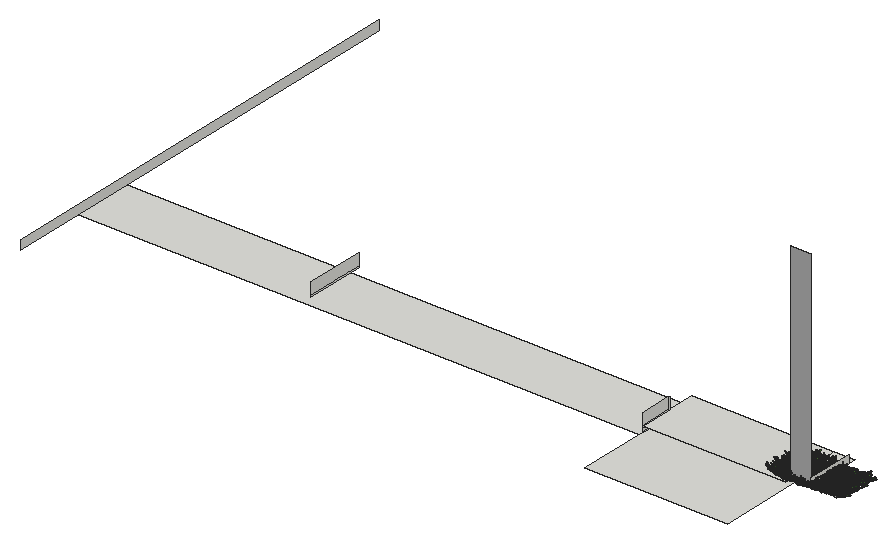
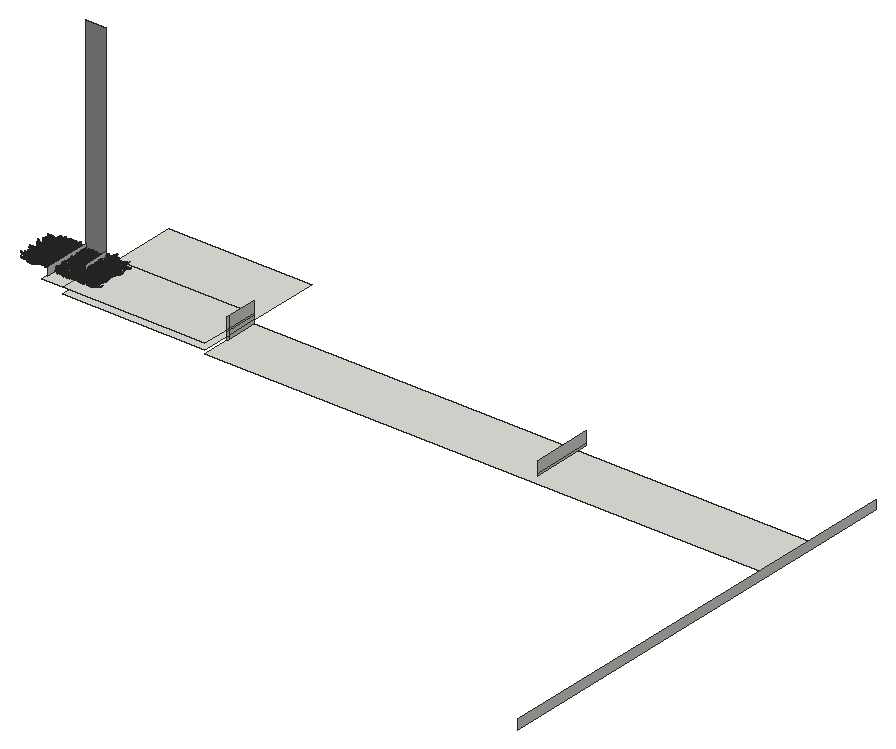
# SketchUp Ruby script. Lengths in inches.
U = 1.inch
M = Sketchup.active_model
def pt(a) = Geom::Point3d.new(a.map { |v| v * U })
def face(e, loops, mat)
  f = e.add_face(loops[0].map { |a| pt(a) })
  loops[1..].each { |l| e.add_face(l.map { |a| pt(a) }).erase! }
  f.material = f.back_material = mat if mat
  f
end
# faces: each face lists its corners as indices into pts; further lists are holes
def faces(e, pts, list, mat = nil) = list.each { |f| face(e, (f[0].is_a?(Array) ? f : [f]).map { |l| l.map { |i| pts[i] } }, mat) }
# xy, xz, yz: faces in a plane at the given z, y or x. An outline is a flat list of corners, or four numbers for a rectangle; further outlines are holes
def ring(l) = l.size == 4 ? [[l[0], l[1]], [l[2], l[1]], [l[2], l[3]], [l[0], l[3]]] : l.each_slice(2).to_a
def flat(e, list, mat, &to3) = list.each { |f| face(e, (f[0].is_a?(Array) ? f : [f]).map { |l| ring(l).map { |u, v| to3.(u, v) } }, mat) }
def xy(e, z, list, mat = nil) = flat(e, list, mat) { |x, y| [x, y, z] }
def xz(e, y, list, mat = nil) = flat(e, list, mat) { |x, z| [x, y, z] }
def yz(e, x, list, mat = nil) = flat(e, list, mat) { |y, z| [x, y, z] }
def lines(e, pts, list) = list.each { |a, b| e.add_line(pt(pts[a]), pt(pts[b])) }
# prism: a flat outline (further loops are holes) pulled along v
def prism(e, loops, v, mat = nil)
  f = face(e, loops, mat); d = Geom::Vector3d.new(v.map { |x| x * U })
  f.pushpull(f.normal.samedirection?(d) ? d.length : -d.length)
end
def box(e, o, s, mat = nil) = prism(e, [[o, [o[0] + s[0], o[1], o[2]], [o[0] + s[0], o[1] + s[1], o[2]], [o[0], o[1] + s[1], o[2]]]], [0, 0, s[2]], mat)
def at(x, y, z, deg = 0) = Geom::Transformation.translation(pt([x, y, z])) * Geom::Transformation.rotation(ORIGIN, Z_AXIS, deg.degrees)
def axes(o, x, y, z) = Geom::Transformation.new([*x, 0, *y, 0, *z, 0, *pt(o).to_a, 1])
def part(name) = M.definitions.add(name)
# library, detail: a bought-in or finely detailed component or shape, given as its bounding box
def library(name, o, s) = part(name).tap { |d| box(d.entities, o, s) }
def detail(e, o, s) = box(e.add_group.entities, o, s)
def put(e, d, t, mat = nil) = e.add_instance(d, t).tap { |i| i.material = mat if mat }
def group(e, t, mat = nil) = e.add_group.tap { |g| g.transformation = t; g.material = mat if mat }.entities
root = M.entities
M.materials.add("Material82").color = [68, 110, 58]
M.materials.add("Material83").color = [48, 90, 38]
M.materials.add("Material84").color = [68, 110, 48]
M.materials.add("Material85").color = [48, 90, 48]
M.materials.add("Material86").color = [58, 110, 58]
M.materials.add("Material87").color = [58, 90, 38]
M.materials.add("Material88").color = [68, 100, 58]
M.materials.add("Material89").color = [48, 100, 38]
M.materials.add("[Color M03]1").color = [170, 170, 170]
c1 = part("grass00")
p = [[-0.6875,0.15,0],[-0.56,0.08,5.52],[-0.04,0.03,2.76],[0.48,-0.02,0],[0.35,-0.02,5.52],[-0.1,-0.14,5.52],
  [-0.12,0.65,8.37],[-0.42,0.65,8.37]]
faces(c1.entities,p,[[0,1,2,3],[3,2,4],[1,5,2],[5,4,2],[1,6,5],[4,5,6],[7,6,1]])
c2 = part("Group16\#1")
put(c2.entities,c1,axes([1.44,-0.61,-0.01],[0.05352,0.12609,0],[-0.10704,0.04543,0.07239],[0.06664,-0.02828,0.11628]),"Material85")
put(c2.entities,c1,axes([0.76,-0.15,-0.01],[0.04676,0.24062,0],[-0.23162,0.04501,0.06642],[0.0652,-0.01267,0.23595]),"Material82")
put(c2.entities,c1,axes([0.79,0.01,-0.01],[-0.00606,0.34651,0],[-0.34381,-0.00602,0.0432],[0.04319,0.00076,0.34386]))
put(c2.entities,c1,axes([1,0.23,-0.01],[-0.07192,0.31144,0],[-0.28722,-0.06632,0.1236],[0.12043,0.02781,0.29478]),"Material84")
put(c2.entities,c1,axes([1.66,0.77,-0.01],[-0.13828,0.29651,0],[-0.21551,-0.1005,0.22471],[0.20365,0.09498,0.23779]),"Material89")
put(c2.entities,c1,axes([0.6875,0.52,-0.01],[-0.18126,0.24051,0],[-0.22746,-0.17142,0.09788],[0.07817,0.05891,0.28481]),"Material84")
put(c2.entities,c1,axes([0.68,0.78,-0.01],[-0.215,0.18688,0],[-0.12385,-0.14248,0.21334],[0.13995,0.16101,0.18878]),"Material82")
put(c2.entities,c1,axes([0.56,1,-0.01],[-0.13756,0.07624,0],[-0.06159,-0.11112,0.0927],[0.04494,0.08108,0.12705]),"Material84")
put(c2.entities,c1,axes([0.2,0.64,-0.01],[-0.23729,0.07254,0],[-0.05711,-0.18681,0.153],[0.04473,0.14632,0.19535]),"Material89")
put(c2.entities,c1,axes([0.0625,0.72,-0.01],[-0.28874,0.02525,0],[-0.02179,-0.24916,0.14647],[0.01276,0.14591,0.25012]),"Material82")
put(c2.entities,c1,axes([-0.08,0.62,-0.01],[-0.34089,-0.04187,0],[0.03255,-0.26504,0.216],[-0.02633,0.21439,0.26703]),"Material89")
put(c2.entities,c1,axes([-0.34,0.98,-0.01],[-0.14314,-0.0493,0],[0.04397,-0.12769,0.06843],[-0.02228,0.0647,0.13505]),"Material89")
put(c2.entities,c1,axes([-0.87,1.45,-0.01],[-0.23488,-0.14114,0],[0.13761,-0.22901,0.06087],[-0.03135,0.05217,0.26717]))
put(c2.entities,c1,axes([-0.72,0.77,-0.01],[-0.14208,-0.13251,0],[0.07209,-0.0773,0.16301],[-0.11118,0.11922,0.1057]),"Material89")
put(c2.entities,c1,axes([-0.62,0.43,-0.01],[-0.14845,-0.21203,0],[0.18654,-0.13061,0.12304],[-0.10079,0.07057,0.22772]),"Material82")
put(c2.entities,c1,axes([-0.68,0.29,-0.01],[-0.13639,-0.32136,0],[0.31723,-0.13464,0.05579],[-0.05136,0.0218,0.34462]),"Material83")
put(c2.entities,c1,axes([-0.64,0.125,-0.01],[-0.0458,-0.23569,0],[0.22124,-0.043,0.08276],[-0.08124,0.01579,0.22538]),"Material86")
put(c2.entities,c1,axes([-1.6,-0.03,-0.01],[0.00576,-0.32897,0],[0.27526,0.00482,0.18018],[-0.18015,-0.00315,0.2753]),"Material84")
put(c2.entities,c1,axes([-1.36,-0.31,-0.01],[0.05718,-0.24765,0],[0.18172,0.04196,0.17267],[-0.16825,-0.03885,0.1865]),"Material89")
put(c2.entities,c1,axes([-1.54,-0.72,-0.01],[0.06537,-0.14017,0],[0.13555,0.06321,0.03939],[-0.0357,-0.01665,0.14956]))
put(c2.entities,c1,axes([-1.19,-0.9,-0.01],[0.09597,-0.12735,0],[0.11214,0.08451,0.07557],[-0.06035,-0.04548,0.14042]),"Material88")
put(c2.entities,c1,axes([-0.47,-0.54,-0.01],[0.11588,-0.10072,0],[0.0618,0.0711,0.12124],[-0.07953,-0.0915,0.0942]))
put(c2.entities,c1,axes([-0.47,-0.84,-0.01],[0.11927,-0.0661,0],[0.06603,0.11913,0.00646],[-0.00313,-0.00565,0.13621]),"Material84")
put(c2.entities,c1,axes([-0.38,-1.24,-0.01],[0.28037,-0.08571,0],[0.0618,0.20215,0.20315],[-0.05939,-0.19428,0.21139]),"Material88")
put(c2.entities,c1,axes([-0.06,-0.66,-0.01],[0.22719,-0.01987,0],[0.01247,0.14255,0.17758],[-0.01547,-0.17691,0.1431]),"Material87")
put(c2.entities,c1,axes([0.11,-0.89,-0.01],[0.14882,0.01828,0],[-0.01058,0.08611,0.12229],[0.01491,-0.12138,0.08676]),"Material85")
put(c2.entities,c1,axes([0.25,-0.72,-0.01],[0.20481,0.07053,0],[-0.06206,0.18022,0.10291],[0.03351,-0.0973,0.1906]),"Material85")
put(c2.entities,c1,axes([0.85,-1.42,-0.01],[0.16481,0.09904,0],[-0.09472,0.15762,0.05616],[0.02893,-0.04814,0.18389]),"Material84")
put(c2.entities,c1,axes([1.01,-1.09,-0.01],[0.21858,0.20385,0],[-0.17495,0.1876,0.15339],[0.10462,-0.11218,0.25652]),"Material89")
put(c2.entities,c1,axes([1.01,-0.71,-0.01],[0.08733,0.12473,0],[-0.06445,0.04512,0.13037],[0.1068,-0.07477,0.07867]),"Material85")
c3 = part("Group15\#1")
put(c3.entities,c2,at(0,0,0))
c4 = part("3darcstudiotree_grass00\#1")
put(c4.entities,c3,at(0,0,0))
xy(root,-42.1875,[[0.34,335.84,486.41,387.84]])
xy(root,-39.125,[[486.41,273.41,609.09,387.84]])
xy(root,-34.17,[[486.41,335.84,609.09,387.84],[609.09,341.03,626.68,387.84]])
xz(root,341.03,[[609.09,-34.17,626.68,144.9375]],"[Color M03]1")
yz(root,0.34,[[273.41,-42.1875,273.41,-38.0625,273.53,-38.0625,273.53,-34.17,659.09,-34.17,659.09,-42.1875]])
yz(root,200.03,[[335.84,-35.625,387.84,-34.17],[335.84,-34.17,387.84,-24.25]])
yz(root,486.41,[[335.84,-42.1875,362.97,-39.125],[362.97,-42.1875,364.46,-39.125],[335.84,-39.125,362.97,-35.625],[362.97,-39.125,364.46,-35.625],[335.84,-35.625,362.97,-34.17],
  [362.97,-35.625,364.46,-34.17],[335.84,-34.17,362.97,-24.25],[362.97,-34.17,364.46,-24.25]])
yz(root,609.09,[[341.03,-34.17,362.97,-27.66]])
yz(root,626.68,[[341.03,-34.17,381.72,-27.66]])
put(root,c4,axes([596.77,350.95,-34.17],[-3.06097,-0.5879,0],[1.66705,-1.34995,-0.03924],[0.1162,-0.0941,1.93013]))
put(root,c4,axes([597.85,372.86,-34.17],[0.43217,-1.5656,0],[4.20709,0.18062,-0.01362],[0.0661,0.00284,1.54899]))
put(root,c4,axes([598.34,355.5625,-34.17],[-4.03652,-0.16228,0],[0.44348,-1.71564,-0.03002],[0.01485,-0.05745,1.59842]))
put(root,c4,axes([598.04,360.35,-34.17],[2.89762,-1.1399,0],[2.43274,0.96179,-0.0036],[0.01556,0.00615,1.5794]))
put(root,c4,axes([597.95,342.71,-34.17],[3.9501,-0.3019,0],[0.82816,1.68526,-0.01483],[0.01308,0.02661,1.51152]))
put(root,c4,axes([597.65,364.46,-34.17],[3.35543,0.83331,0],[-2.02345,1.2672,-0.03908],[-0.13338,0.08353,1.82303]))
put(root,c4,axes([598.39,348.62,-34.17],[2.855,1.42821,0],[-2.79418,0.86872,-0.04305],[-0.19263,0.05989,1.51958]))
put(root,c4,axes([600.08,371.03,-34.17],[4.14496,0.31804,0],[-0.83759,1.6978,-0.03864],[-0.04159,0.0843,1.85268]))
put(root,c4,axes([600.26,342.22,-34.17],[3.14768,1.20624,0],[-3.13864,1.27383,-0.06236],[-0.23969,0.09728,1.86199]))
put(root,c4,axes([601.58,367.78,-34.17],[1.22629,-1.22817,0],[3.78204,0.58732,-0.0431],[0.18193,0.02825,1.38217]))
put(root,c4,axes([601.63,354.84,-34.17],[2.09831,-1.02697,0],[3.53268,1.1226,-0.04335],[0.15343,0.04876,1.54559]))
put(root,c4,axes([601.5,351.3,-34.17],[-2.72452,1.24598,0],[-3.55259,-1.2082,-0.04683],[-0.18808,-0.06396,1.86493]))
put(root,c4,axes([600.98,357.3125,-34.17],[3.77194,0.53127,0],[-1.56854,1.73204,-0.02984],[-0.04464,0.0493,1.55474]))
put(root,c4,axes([602.62,353.18,-34.17],[0.71144,-1.32945,0],[4.31841,0.35942,-0.04294],[0.17046,0.01419,1.34209]))
put(root,c4,axes([602.9,360.26,-34.17],[1.7149,-1.22637,0],[3.67075,0.79833,-0.00061],[0.00329,0.00072,1.94394]))
put(root,c4,axes([603.23,362.27,-34.17],[1.13517,-1.33714,0],[4.08386,0.53922,-0.04023],[0.16123,0.02129,1.36415]))
put(root,c4,axes([602.3125,366.27,-34.17],[-1.96155,1.42232,0],[-3.86474,-0.82896,-0.01158],[-0.04562,-0.00979,1.47884]))
put(root,c4,axes([603.71,372.46,-34.17],[-0.47401,-1.83018,0],[3.81106,-0.15352,-0.01024],[0.06486,-0.00261,1.82793]))
put(root,c4,axes([603.14,363.91,-34.17],[-2.22727,1.60419,0],[-4.12877,-0.89155,-0.00813],[-0.02667,-0.00576,1.31962]))
put(root,c4,axes([603.48,348.36,-34.17],[-2.60888,1.40075,0],[-3.4553,-1.0009,-0.02364],[-0.11495,-0.0333,1.93862]))
put(root,c4,axes([603.86,347.26,-34.17],[3.43972,-1.19732,0],[3.07284,1.37298,-0.00351],[0.01073,0.00479,1.60808]))
put(root,c4,axes([603.88,344.94,-34.17],[2.57433,-1.10368,0],[3.03991,1.10279,-0.05921],[0.27011,0.09799,1.91907]))
put(root,c4,axes([605.8,364.41,-34.17],[-1.00872,-1.50256,0],[3.76018,-0.39261,-0.00114],[0.00668,-0.0007,1.77079]))
put(root,c4,axes([606.1,351.03,-34.17],[-4.39065,-0.68044,0],[1.48247,-1.48779,-0.03326],[0.06181,-0.06203,1.54402]))
put(root,c4,axes([606.08,365.79,-34.17],[-4.44259,0.07323,0],[-0.15396,-1.45277,-0.02048],[-0.00618,-0.05831,1.99696]))
put(root,c4,axes([605.59,361.58,-34.17],[-2.76199,0.84111,0],[-2.40625,-1.22891,-0.02049],[-0.06035,-0.03082,1.42185]))
put(root,c4,axes([606.19,344.48,-34.17],[4.22079,-0.16227,0],[0.44484,1.79962,-0.00515],[0.00263,0.01065,1.80879]))
put(root,c4,axes([608.31,341.46,-34.17],[-4.16244,-0.15093,0],[0.36502,-1.56574,-0.01686],[0.00714,-0.03063,1.38194]))
put(root,c4,axes([606.99,358.125,-34.17],[-0.6643,1.32662,0],[-4.47997,-0.3489,-0.01512],[-0.08059,-0.00628,1.85999]))
put(root,c4,axes([608.55,349.27,-34.17],[0.943,-1.41783,0],[3.80413,0.39351,-0.01105],[0.05525,0.00572,1.52421]))
put(root,c4,axes([607.11,340.13,-34.17],[0.93193,1.68006,0],[-3.63506,0.3136,-0.00261],[-0.01526,0.00132,1.6704]))
put(root,c4,axes([609.1875,355.56,-34.17],[-3.93808,-0.75827,0],[2.05575,-1.66052,-0.06565],[0.13947,-0.11266,1.70067]))
put(root,c4,axes([607.58,359.26,-34.17],[-0.07538,1.68656,0],[-4.43832,-0.03085,-0.00958],[-0.0427,-0.0003,1.48335]))
put(root,c4,axes([608.42,347.11,-34.17],[0.31598,1.50106,0],[-3.48689,0.11416,-0.00998],[-0.05116,0.00168,1.34846]))
put(root,c4,axes([609.24,371.18,-34.17],[3.02082,-1.15648,0],[2.42176,0.98385,-0.02978],[0.11407,0.04634,1.43312]))
put(root,c4,axes([608.69,367.64,-34.17],[3.58704,0.55594,0],[-1.39662,1.40151,-0.02634],[-0.05335,0.05353,1.58474]))
put(root,c4,axes([609.32,352.21,-34.17],[3.13564,-0.95157,0],[2.13614,1.09478,-0.03629],[0.11919,0.06109,1.41389]))
put(root,c4,axes([611.19,369.84,-34.17],[-3.8239,-0.32025,0],[0.87863,-1.63166,-0.02543],[0.02678,-0.04974,1.60712]))
put(root,c4,axes([611.99,364.32,-34.17],[-1.37854,-1.47975,0],[3.2131,-0.46555,-0.02344],[0.115,-0.01666,1.34096]))
put(root,c4,axes([611.77,346.58,-34.17],[-3.58928,0.33039,0],[-0.75882,-1.28211,-0.0198],[-0.02657,-0.04489,1.47686]))
put(root,c4,axes([611.6,366.04,-34.17],[1.03001,-1.55898,0],[3.46185,0.35573,-0.04641],[0.24674,0.02535,1.47323]))
put(root,c4,axes([612.35,361.51,-34.17],[0.07037,-1.71405,0],[4.70144,0.03002,-0.02796],[0.12644,0.00081,1.59394]))
put(root,c4,axes([612.45,358.96,-34.17],[-4.25189,0.62806,0],[-1.17044,-1.23238,-0.01358],[-0.02814,-0.02963,1.47772]))
put(root,c4,axes([612.82,357.41,-34.17],[-4.15804,-0.01553,0],[0.04454,-1.85443,-0.04475],[0.00172,-0.0718,1.43393]))
put(root,c4,axes([612.16,373.13,-34.17],[2.99211,-0.88341,0],[2.54027,1.33816,-0.01707],[0.06311,0.03325,1.96039]))
put(root,c4,axes([613.01,355.67,-34.17],[-3.68076,-0.30441,0],[0.87866,-1.65237,-0.00999],[0.00884,-0.01661,1.38276]))
put(root,c4,axes([612.66,369.11,-34.17],[-2.36198,1.34531,0],[-2.91809,-0.79683,-0.03104],[-0.17128,-0.04677,1.78553]))
put(root,c4,axes([613.125,344.33,-34.17],[2.97125,-1.188,0],[2.63587,1.02532,-0.00165],[0.00768,0.00299,1.81884]))
put(root,c4,axes([614.28,341.39,-34.17],[-4.35861,-0.14504,0],[0.36663,-1.71363,-0.02802],[0.01298,-0.06068,1.8014]))
put(root,c4,axes([612.98,352.64,-34.17],[3.6615,0.00284,0],[-0.00662,1.32579,-0.0306],[-0.00046,0.09111,1.9022]))
put(root,c4,axes([614.39,351.26,-34.17],[-3.40532,-0.07402,0],[0.22612,-1.61806,-0.00601],[0.00193,-0.01379,1.79325]))
put(root,c4,axes([613.38,349.14,-34.17],[3.15923,1.14894,0],[-3.00225,1.28393,-0.03053],[-0.12215,0.05224,1.95907]))
put(root,c4,axes([616.42,341.86,-34.17],[3.82244,-0.70635,0],[1.81239,1.52539,-0.00986],[0.01787,0.01504,1.36783]))
put(root,c4,axes([617.38,359.25,-34.17],[-3.50881,1.16011,0],[-2.69176,-1.26622,-0.04843],[-0.14054,-0.06611,1.41858]))
put(root,c4,axes([616.77,353.67,-34.17],[3.5983,-0.42057,0],[0.96573,1.28508,-0.03127],[0.05191,0.06908,1.48816]))
put(root,c4,axes([616.78,351.11,-34.17],[-1.39865,1.66077,0],[-3.78259,-0.49545,-0.00679],[-0.0282,-0.00369,1.30662]))
put(root,c4,axes([617.58,364.09,-34.17],[2.65926,-1.384,0],[3.07673,0.91944,-0.04967],[0.23773,0.07104,1.73743]))
put(root,c4,axes([616.96,346.05,-34.17],[3.23293,0.85538,0],[-2.19162,1.28829,-0.0468],[-0.14196,0.08345,1.60535]))
put(root,c4,axes([618.6875,373.03,-34.17],[0.37423,-1.77165,0],[3.6892,0.1212,-0.04948],[0.31334,0.01029,1.76318]))
put(root,c4,axes([618.08,370.58,-34.17],[-1.23102,1.43236,0],[-4.00109,-0.53481,-0.05878],[-0.24424,-0.03265,1.38915]))
put(root,c4,axes([619.35,368.61,-34.17],[-3.85586,-0.61181,0],[1.38378,-1.3564,-0.02256],[0.04705,-0.04612,1.55256]))
put(root,c4,axes([617.87,365.61,-34.17],[4.58666,-0.29954,0],[0.76961,1.83286,-0.06031],[0.05541,0.13196,1.9859]))
put(root,c4,axes([617.58,356.65,-34.17],[2.59618,1.43862,0],[-2.87173,0.80602,-0.01154],[-0.04691,0.01317,1.31865]))
put(root,c4,axes([619.11,344.33,-34.17],[0.50435,-1.60129,0],[3.80498,0.18639,-0.05019],[0.26525,0.01299,1.53052]))
put(root,c4,axes([618.4,362.3,-34.17],[3.24935,0.42764,0],[-1.43334,1.69386,-0.04175],[-0.05922,0.06999,1.52086]))
put(root,c4,axes([618.77,348.15,-34.17],[4.09406,-0.23131,0],[0.47213,1.29969,-0.032],[0.03631,0.09996,1.99674]))
put(root,c4,axes([619.21,340.25,-34.17],[1.78223,1.25772,0],[-3.10123,0.68348,-0.02391],[-0.11693,0.02577,1.49173]))
put(root,c4,axes([619.22,355.03,-34.17],[0.65139,1.7147,0],[-4.45072,0.26296,-0.01905],[-0.08769,0.00518,1.57029]))
put(root,c4,axes([622.5,370.89,-34.17],[-3.04991,-1.12114,0],[2.90905,-1.23081,-0.00052],[0.00199,-0.00084,1.79691]))
put(root,c4,axes([624.15,368.53,-34.17],[0.23876,-1.55199,0],[4.36064,0.10434,-0.04584],[0.18368,0.0044,1.3146]))
put(root,c4,axes([624.41,351.125,-34.17],[-0.00481,-1.55543,0],[4.64446,-0.00224,-0.02113],[0.08601,-0.00004,1.41674]))
put(root,c4,axes([623.08,344.05,-34.17],[3.47227,-0.30693,0],[0.74979,1.31925,-0.01015],[0.01336,0.0235,1.54623]))
put(root,c4,axes([623.05,346.05,-34.17],[-1.26342,1.38148,0],[-3.54227,-0.50384,-0.00809],[-0.04856,-0.00691,1.80065]))
put(root,c4,axes([623.6875,352.72,-34.17],[2.94151,-0.90679,0],[2.69176,1.35804,-0.00613],[0.02014,0.01016,1.74641]))
put(root,c4,axes([622.95,365.35,-34.17],[0.11831,1.37685,0],[-3.50344,0.04682,-0.00216],[-0.01444,0.00019,1.758]))
put(root,c4,axes([624.61,356.01,-34.17],[-0.73982,-1.44093,0],[3.74487,-0.29904,-0.04711],[0.2431,-0.01941,1.50792]))
put(root,c4,axes([624.1,361.35,-34.17],[2.48182,-1.04217,0],[2.75852,1.02169,-0.02466],[0.10108,0.03744,1.59511]))
put(root,c4,axes([623.93,348.7,-34.17],[-2.81085,1.01922,0],[-2.91901,-1.25203,-0.0061],[-0.02341,-0.01004,1.83281]))
put(root,c4,axes([623.87,341.63,-34.17],[-0.96185,1.4826,0],[-3.70839,-0.37418,-0.04208],[-0.21883,-0.02208,1.54007]))
put(root,c4,axes([625.34,359.52,-34.17],[-0.3225,-1.34219,0],[4.58247,-0.17125,-0.03587],[0.16603,-0.0062,1.60406]))
put(root,c4,axes([624.07,340.65,-34.17],[3.91343,0.66663,0],[-1.38696,1.26634,-0.02193],[-0.04877,0.04453,1.47013]))
put(root,c4,axes([624.88,363.84,-34.17],[3.82293,-1.07301,0],[2.00012,1.10831,-0.02041],[0.08948,0.04958,1.95445]))
put(root,c4,axes([624.75,357.49,-34.17],[3.70183,0.03147,0],[-0.07805,1.42775,-0.0399],[-0.00598,0.10931,1.8861]))
put(root,c4,axes([628.43,354.69,-34.17],[-0.79677,-1.6402,0],[3.36468,-0.25421,-0.01579],[0.08769,-0.00662,1.45182]))
put(root,c4,axes([628.94,350.28,-34.17],[-4.49567,-0.3985,0],[0.83225,-1.46029,-0.03373],[0.03467,-0.06083,1.33323]))
put(root,c4,axes([628.86,352.49,-34.17],[-4.6805,0.28538,0],[-0.54089,-1.37973,-0.03554],[-0.03758,-0.09587,1.83631]))
put(root,c4,axes([627.59,358.97,-34.17],[-0.10316,1.55622,0],[-4.09748,-0.04224,-0.03889],[-0.19104,-0.00197,1.50954]))
put(root,c4,axes([628.4,356.86,-34.17],[-3.29804,1.27107,0],[-2.52678,-1.01968,-0.01484],[-0.07094,-0.02863,1.85373]))
put(root,c4,axes([628.53,363.52,-34.17],[2.48968,-1.1461,0],[2.93182,0.99053,-0.00664],[0.0258,0.00872,1.48048]))
put(root,c4,axes([629.98,368.03,-34.17],[-1.20508,-1.27416,0],[3.97727,-0.58504,-0.0406],[0.22085,-0.03249,1.84742]))
put(root,c4,axes([629.125,346.98,-34.17],[-0.56456,1.41966,0],[-3.50259,-0.21664,-0.01794],[-0.10644,-0.00658,1.59592]))
put(root,c4,axes([629.1,366.93,-34.17],[1.96349,1.64722,0],[-3.56633,0.66117,-0.03464],[-0.18907,0.03505,1.78143]))
put(root,c4,axes([630.91,361.32,-34.17],[2.10633,-1.56652,0],[4.07545,0.85227,-0.05067],[0.19625,0.04104,1.51576]))
put(root,c4,axes([630.82,341.8,-34.17],[2.08347,-1.59715,0],[3.15506,0.64012,-0.03693],[0.21917,0.04447,1.77491]))
put(root,c4,axes([629.86,348.7,-34.17],[0.79004,1.45858,0],[-4.26548,0.35933,-0.00171],[-0.00893,0.00075,1.74655]))
put(root,c4,axes([631.58,371.06,-34.17],[1.69514,-1.26112,0],[3.85825,0.80658,-0.01977],[0.09529,0.01992,1.78562]))
put(root,c4,axes([630.44,343.68,-34.17],[3.33408,0.32893,0],[-1.10916,1.74856,-0.00744],[-0.00738,0.01164,1.4009]))
put(root,c4,axes([634.15,348.7,-34.17],[-4.09965,-0.15274,0],[0.36855,-1.53851,-0.03137],[0.01329,-0.05547,1.3228]))
put(root,c4,axes([633.6,366.12,-34.17],[-3.21191,1.28173,0],[-2.59769,-1.01243,-0.03007],[-0.15402,-0.06003,1.97134]))
put(root,c4,axes([634.6,356.73,-34.17],[-1.51918,-1.57572,0],[4.39344,-0.65879,-0.02869],[0.10716,-0.01607,1.40786]))
put(root,c4,axes([634.97,341.9,-34.17],[-4.22007,0.35003,0],[-0.86715,-1.62599,-0.01674],[-0.0198,-0.03713,1.81501]))
put(root,c4,axes([634.34,361.08,-34.17],[-1.69964,1.49974,0],[-3.25198,-0.57319,-0.0353],[-0.21623,-0.03811,1.79152]))
put(root,c4,axes([634.31,360.03,-34.17],[-1.65501,1.23077,0],[-2.99443,-0.62625,-0.02105],[-0.13776,-0.02881,1.88169]))
put(root,c4,axes([633.64,346.7,-34.17],[3.27704,0.72692,0],[-1.98468,1.39155,-0.00275],[-0.00611,0.00428,1.37565]))
put(root,c4,axes([635.58,350.27,-34.17],[-2.87872,-0.88154,0],[2.80816,-1.42624,-0.06125],[0.14894,-0.07565,1.36064]))
put(root,c4,axes([635.13,355.28,-34.17],[0.11814,-1.8536,0],[3.92163,0.03887,-0.05528],[0.30038,0.00298,1.59813]))
put(root,c4,axes([636.49,364.48,-34.17],[-1.1098,-1.31734,0],[3.29231,-0.43138,-0.00285],[0.02011,-0.00264,1.93438]))
put(root,c4,axes([636.46,353.16,-34.17],[-2.16844,-1.41891,0],[2.90956,-0.69156,-0.03107],[0.17396,-0.04135,1.66455]))
put(root,c4,axes([636.69,369.03,-34.17],[-3.85239,-0.20163,0],[0.58764,-1.74619,-0.01228],[0.0079,-0.02349,1.63767]))
put(root,c4,axes([636.74,370.22,-34.17],[-1.66799,1.12199,0],[-3.57556,-0.82672,-0.01566],[-0.07039,-0.01628,1.61828]))
put(root,c4,axes([636.84,344.16,-34.17],[3.70469,-0.86578,0],[1.68851,1.12372,-0.02001],[0.07058,0.04697,1.71774]))
put(root,c4,axes([641.17,369.12,-34.17],[-4.16983,-0.88311,0],[1.85574,-1.3628,-0.02099],[0.05036,-0.03698,1.49075]))
put(root,c4,axes([640.4,351.28,-34.17],[2.24844,-1.02464,0],[3.26531,1.11441,-0.03846],[0.14191,0.04843,1.57923]))
put(root,c4,axes([641.15,370.01,-34.17],[-1.93961,-1.1589,0],[2.81158,-0.73187,-0.03406],[0.19491,-0.05074,1.73123]))
put(root,c4,axes([641.51,348.88,-34.17],[-2.17228,-1.46024,0],[3.41853,-0.79094,-0.03431],[0.15337,-0.03548,1.53951]))
put(root,c4,axes([640.84,361.59,-34.17],[2.63669,-1.45672,0],[3.66232,1.03098,-0.04124],[0.15536,0.04373,1.56101]))
put(root,c4,axes([640.34,360.14,-34.17],[3.40582,0.10745,0],[-0.34866,1.71886,-0.00093],[-0.00031,0.0015,1.35201]))
put(root,c4,axes([640.06,346.68,-34.17],[4.00271,0.72936,0],[-1.54017,1.31459,-0.00765],[-0.0159,0.01357,1.36419]))
put(root,c4,axes([641.89,365.68,-34.17],[0.50947,-1.51274,0],[4.49668,0.23554,-0.03191],[0.15996,0.00838,1.71939]))
put(root,c4,axes([642.14,342.24,-34.17],[-4.17152,-0.5223,0],[1.23744,-1.53711,-0.0262],[0.03523,-0.04376,1.36239]))
put(root,c4,axes([642.13,354.41,-34.17],[-3.49855,-0.51529,0],[1.58914,-1.67809,-0.03885],[0.07118,-0.07517,1.78292]))
put(root,c4,axes([640.4,363.2,-34.17],[-0.28743,1.31478,0],[-4.42266,-0.15037,-0.00545],[-0.03167,-0.00108,1.93955]))
put(root,c4,axes([642.55,356.97,-34.17],[-3.86459,-0.0799,0],[0.17825,-1.34085,-0.00586],[0.00206,-0.0155,1.71352]))
put(root,c4,axes([641.13,353.04,-34.17],[0.76665,1.71699,0],[-3.34963,0.23261,-0.02162],[-0.1104,0.00767,1.32159]))
put(root,c4,axes([642.39,344.93,-34.17],[3.46997,0.08994,0],[-0.27266,1.63611,-0.01423],[-0.00549,0.03292,1.83161]))
put(root,c4,axes([644.64,342.63,-34.17],[-4.50934,-0.15911,0],[0.38591,-1.70103,-0.03473],[0.01636,-0.07211,1.7157]))
put(root,c4,axes([645.32,356.79,-34.17],[-1.29023,-1.58759,0],[3.9469,-0.49888,-0.03893],[0.19606,-0.02478,1.64312]))
put(root,c4,axes([645.58,359.51,-34.17],[-3.37238,-1.2695,0],[3.05865,-1.2637,-0.04863],[0.19789,-0.08176,1.95701]))
put(root,c4,axes([645.32,368.54,-34.17],[0.71095,-1.43364,0],[4.62721,0.35689,-0.06032],[0.23627,0.01822,1.41053]))
put(root,c4,axes([645.36,362.16,-34.17],[-3.5162,-0.01544,0],[0.03762,-1.33225,-0.02017],[0.00158,-0.05579,1.77597]))
put(root,c4,axes([645.91,344.06,-34.17],[-2.35898,-1.49879,0],[3.37563,-0.82632,-0.02087],[0.09435,-0.0231,1.58468]))
put(root,c4,axes([645.04,349.125,-34.17],[2.33704,1.50763,0],[-2.98263,0.71909,-0.02868],[-0.14145,0.0341,1.51486]))
put(root,c4,axes([646.86,372.63,-34.17],[-0.8203,-1.58295,0],[4.36315,-0.35165,-0.03636],[0.17472,-0.01408,1.63697]))
put(root,c4,axes([647.7,347.07,-34.17],[0.6786,-1.83556,0],[4.57598,0.26311,-0.00277],[0.01184,0.00068,1.49508]))
put(root,c4,axes([646.21,369.6875,-34.17],[3.70622,-0.07941,0],[0.19617,1.42399,-0.02262],[0.0073,0.05302,1.6131]))
put(root,c4,axes([646.34,350.86,-34.17],[2.20491,1.1875,0],[-2.92266,0.84401,-0.01948],[-0.09978,0.02881,1.72408]))
put(root,c4,axes([647.9,364.14,-34.17],[-3.77729,0.83126,0],[-1.83032,-1.29355,-0.03544],[-0.09552,-0.06751,1.55733]))
put(root,c4,axes([647.99,354.53,-34.17],[1.99944,-1.04992,0],[3.08282,0.91308,-0.00267],[0.01382,0.00409,1.87177]))
